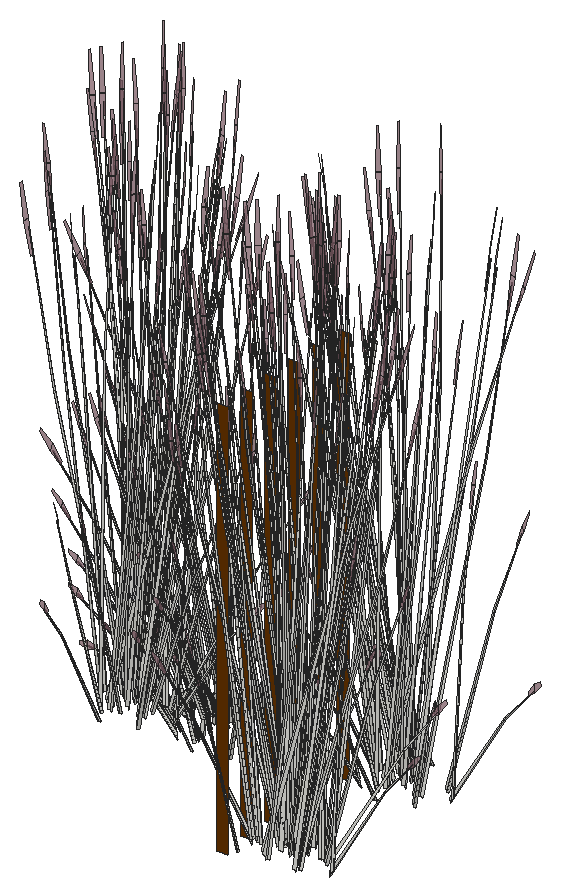
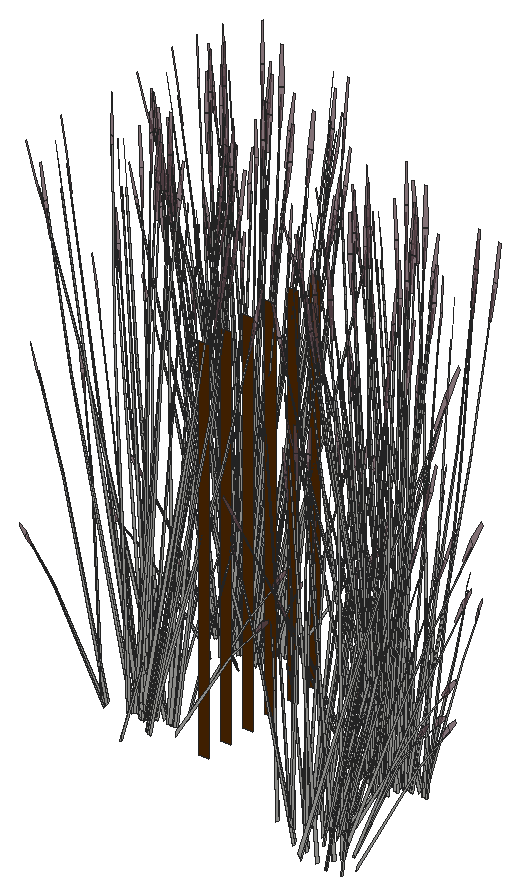
# SketchUp Ruby script. Lengths in inches.
U = 1.inch
M = Sketchup.active_model
def pt(a) = Geom::Point3d.new(a.map { |v| v * U })
def face(e, loops, mat)
  f = e.add_face(loops[0].map { |a| pt(a) })
  loops[1..].each { |l| e.add_face(l.map { |a| pt(a) }).erase! }
  f.material = f.back_material = mat if mat
  f
end
# faces: each face lists its corners as indices into pts; further lists are holes
def faces(e, pts, list, mat = nil) = list.each { |f| face(e, (f[0].is_a?(Array) ? f : [f]).map { |l| l.map { |i| pts[i] } }, mat) }
# xy, xz, yz: faces in a plane at the given z, y or x. An outline is a flat list of corners, or four numbers for a rectangle; further outlines are holes
def ring(l) = l.size == 4 ? [[l[0], l[1]], [l[2], l[1]], [l[2], l[3]], [l[0], l[3]]] : l.each_slice(2).to_a
def flat(e, list, mat, &to3) = list.each { |f| face(e, (f[0].is_a?(Array) ? f : [f]).map { |l| ring(l).map { |u, v| to3.(u, v) } }, mat) }
def xy(e, z, list, mat = nil) = flat(e, list, mat) { |x, y| [x, y, z] }
def xz(e, y, list, mat = nil) = flat(e, list, mat) { |x, z| [x, y, z] }
def yz(e, x, list, mat = nil) = flat(e, list, mat) { |y, z| [x, y, z] }
def lines(e, pts, list) = list.each { |a, b| e.add_line(pt(pts[a]), pt(pts[b])) }
# prism: a flat outline (further loops are holes) pulled along v
def prism(e, loops, v, mat = nil)
  f = face(e, loops, mat); d = Geom::Vector3d.new(v.map { |x| x * U })
  f.pushpull(f.normal.samedirection?(d) ? d.length : -d.length)
end
def box(e, o, s, mat = nil) = prism(e, [[o, [o[0] + s[0], o[1], o[2]], [o[0] + s[0], o[1] + s[1], o[2]], [o[0], o[1] + s[1], o[2]]]], [0, 0, s[2]], mat)
def at(x, y, z, deg = 0) = Geom::Transformation.translation(pt([x, y, z])) * Geom::Transformation.rotation(ORIGIN, Z_AXIS, deg.degrees)
def axes(o, x, y, z) = Geom::Transformation.new([*x, 0, *y, 0, *z, 0, *pt(o).to_a, 1])
def part(name) = M.definitions.add(name)
# library, detail: a bought-in or finely detailed component or shape, given as its bounding box
def library(name, o, s) = part(name).tap { |d| box(d.entities, o, s) }
def detail(e, o, s) = box(e.add_group.entities, o, s)
def put(e, d, t, mat = nil) = e.add_instance(d, t).tap { |i| i.material = mat if mat }
def group(e, t, mat = nil) = e.add_group.tap { |g| g.transformation = t; g.material = mat if mat }.entities
root = M.entities
M.materials.add("C08_Toffee_Ember").color = [102, 51, 0]
M.materials.add("LightPink_Translucent").color = [144, 107, 117]
M.materials["LightPink_Translucent"].alpha = 0.75
c1 = part("blade")
p = [[2.15,0.21,22],[0,0.17,0],[0.09,0.45,0],[2.18,0.31,22],[2.29,0.31,22],[0.38,0.45,0],
  [2.48,0.24,33],[2.49,0.24,33],[2.48,0.22,33]]
faces(c1.entities,p,[[0,1,2,3],[4,5,2,3],[6,3,4,7],[8,0,3,6]])
c2 = part("seeds")
p = [[0.3,-0.1,1.38],[-0.01,-0.03,1.59],[-0.01,-0.03,0.03],[0.14,-0.07,-0.07],[0.29,-0.03,3],[0.15,0.01,3.11]]
faces(c2.entities,p,[[0,1,2,3],[1,0,4,5]],"LightPink_Translucent")
c3 = part("blade with seeds")
put(c3.entities,c1,at(0,0,0))
put(c3.entities,c2,axes([2.4,0.25,30.99],[1.5799,-0.05474,1.17369],[-0.12525,1.92788,0.29478],[-0.07173,-0.02425,1.56792]))
xz(root,322.2,[[693.41,510,694.41,546]],"C08_Toffee_Ember")
xz(root,324.9,[[693.41,510,694.41,546]],"C08_Toffee_Ember")
xz(root,327.6,[[693.41,510,694.41,546]],"C08_Toffee_Ember")
xz(root,330.3,[[693.41,510,694.41,546]],"C08_Toffee_Ember")
xz(root,333,[[693.41,510,694.41,546]],"C08_Toffee_Ember")
xz(root,335.7,[[693.41,510,694.41,546]],"C08_Toffee_Ember")
put(root,c3,axes([697.01,322.31,511.68],[0.45414,-0.35624,-0.25712],[0.45414,0.35624,0.25712],[0,-0.11474,1.15348]))
put(root,c3,axes([696.82,320.6,511.77],[-0.18768,0.46622,-0.03231],[-0.57763,-0.14342,-0.14649],[-0.0877,-0.07626,0.48318]))
put(root,c3,axes([698.6,322.96,512.21],[-0.73268,-0.27244,-0.24149],[0.35279,-0.57501,-0.41502],[-0.02303,-0.14118,1.32557]))
put(root,c3,axes([696.51,322.73,511.97],[-0.81352,0,0],[0,-0.63814,-0.42834],[0,-0.14534,1.3588]))
put(root,c3,axes([698.86,320.83,511.68],[0.60696,0.14127,-0.25712],[-0.15283,0.49751,0.25712],[0.12236,-0.05737,1.15348]))
put(root,c3,axes([697.14,322.56,511.93],[-0.60515,0.48003,0.25528],[-0.60552,-0.47498,-0.30288],[-0.02113,-0.13632,1.36855]))
put(root,c3,axes([699.07,322.78,512.02],[0.73304,0.27674,0.19974],[-0.35279,0.57501,0.41502],[0,-0.13255,1.3325]))
put(root,c3,axes([698.78,323.56,512.02],[0.17244,-0.67657,-0.19446],[0.81759,0.11793,0.42555],[-0.14286,-0.09343,1.29846]))
put(root,c3,axes([701.16,320.84,511.97],[0.40676,-0.57214,0],[0.68052,0.31907,-0.42834],[0.15499,0.07267,1.3588]))
put(root,c3,axes([698.72,323.29,511.83],[-0.39083,-0.47924,-0.37133],[0.59199,-0.33747,0.17871],[-0.12647,-0.0593,1.19224]))
put(root,c3,axes([698.8,322.61,511.96],[0.28286,0.63846,0.37976],[-0.80821,0.22202,0.14902],[0.00988,-0.11732,1.31851]))
put(root,c3,axes([702.76,323.1,511.65],[-0.41902,0.06852,1.17514],[-0.0667,-0.54541,0.06726],[0.29348,-0.08255,0.6687]))
put(root,c3,axes([703.52,322.62,511.875],[-0.40335,-0.3651,-0.05385],[0.44175,-0.33453,-0.24415],[0.12517,-0.02355,0.8053]))
put(root,c3,axes([699.82,322.66,511.83],[0,-0.66065,0],[0.81352,0,0],[0,0,1.48949]))
put(root,c3,axes([698.37,323.47,511.71],[-0.67676,-0.09361,-0.51753],[0.14281,-0.57742,-0.13583],[-0.20196,-0.06997,1.14236]))
put(root,c3,axes([699.4375,322.25,511.96],[-0.53943,0.51816,0.37976],[-0.64086,-0.4574,0.14902],[0.13005,-0.05171,1.31851]))
put(root,c3,axes([700.03,323.17,511.91],[-0.60515,-0.49144,-0.05089],[0.60552,-0.49174,0],[-0.02113,-0.01716,1.45724]))
put(root,c3,axes([698.22,321.85,511.32],[-0.64037,0.22859,1.07011],[-0.20382,-0.65589,0.4158],[0.39323,0.01091,1.21713]))
put(root,c3,axes([699.9375,322.02,512.17],[0.12551,-0.50956,0.12018],[0.6132,0.08845,-0.34318],[0.1116,0.05232,1.05198]))
put(root,c3,axes([698.875,323.23,511.96],[0.82229,0.1203,0.37976],[-0.16734,0.67942,0.14902],[-0.12017,-0.06561,1.31851]))
put(root,c3,axes([703.22,322.74,511.24],[-0.034,-0.08668,1.46364],[0.23582,-0.50706,-0.2236],[0.23788,-0.00729,0.24931]))
put(root,c3,axes([696.2,322.65,511.24],[0.0165,0.08998,1.46364],[-0.33262,0.46992,-0.2236],[-0.23626,-0.02369,0.24931]))
put(root,c3,axes([697.65,324.35,511.68],[-0.15283,-0.49751,-0.25712],[0.60696,-0.14127,0.25712],[-0.12236,-0.05737,1.15348]))
put(root,c3,axes([699.875,322.1875,512.21],[0.65687,-0.37907,-0.24149],[0.43681,0.53562,-0.41502],[0.16207,0.0544,1.32557]))
put(root,c3,axes([697.48,324.5625,511.67],[-0.60889,-0.28548,-0.4121],[0.36394,-0.51192,0],[-0.13868,-0.06502,1.30728]))
put(root,c3,axes([701.53,321.18,511.67],[0.60889,0.28548,-0.4121],[-0.36394,0.51192,0],[0.13868,0.06502,1.30728]))
put(root,c3,axes([700.375,322.81,511.83],[0.72788,0,0],[0,0.59111,0],[0,0,1.48078]))
put(root,c3,axes([699.14,323.55,512.21],[-0.65687,0.37907,-0.24149],[-0.43681,-0.53562,-0.41502],[-0.16207,-0.0544,1.32557]))
put(root,c3,axes([701.36,321.39,511.68],[0.15283,0.49751,-0.25712],[-0.60696,0.14127,0.25712],[0.12236,0.05737,1.15348]))
put(root,c3,axes([700.14,322.51,511.98],[-0.82229,-0.1203,0.40835],[0.16734,-0.67942,0.16024],[0.12017,0.06561,1.41775]))
put(root,c3,axes([699.48,324.1875,511.83],[-0.21227,-0.49226,0],[0.60616,-0.17239,0],[0,0,1.28128]))
put(root,c3,axes([699.08,323.72,512.17],[-0.12551,0.50956,0.12018],[-0.6132,-0.08845,-0.34318],[-0.1116,-0.05232,1.05198]))
put(root,c3,axes([700.28,324.12,511.8125],[0.68303,-0.19373,-0.15934],[0.24001,0.55805,0.00007],[0.07539,-0.02141,1.44335]))
put(root,c3,axes([700.36,323.0625,511.84],[0.45414,0.3688,0],[-0.45414,0.3688,0],[0,0,1.40491]))
put(root,c3,axes([700.64,322.27,511.71],[0.67676,0.09361,-0.51753],[-0.14281,0.57742,-0.13583],[0.20196,0.06997,1.14236]))
put(root,c3,axes([699.33,324.41,511.82],[-0.65588,-0.25634,0],[0.31565,-0.53263,0],[0,0,1.35047]))
put(root,c3,axes([699.88,323.73,512.05],[-0.63528,-0.45956,-0.20909],[0.53456,-0.51604,0.45758],[-0.17107,0.05376,1.39619]))
put(root,c3,axes([700.23,322.93,511.9],[0,0.66033,-0.04679],[-0.81352,0,0],[0,0.02075,1.48875]))
put(root,c3,axes([700.29,322.46,511.83],[0.39083,0.47924,-0.37133],[-0.59199,0.33747,0.17871],[0.12647,0.0593,1.19224]))
put(root,c3,axes([697.86,324.91,511.97],[-0.40676,0.57214,0],[-0.68052,-0.31907,-0.42834],[-0.15499,-0.07267,1.3588]))
put(root,c3,axes([700.625,322.75,512.17],[0.60616,-0.16651,0.12018],[0.21227,0.47548,-0.34318],[0,0.10465,1.05198]))
put(root,c3,axes([699.56,323.63,511.83],[-0.70648,0.03525,-0.37133],[-0.06389,-0.58508,0.17871],[-0.12647,0.0593,1.19224]))
put(root,c3,axes([700.08,324.42,511.83],[0.65588,0.25634,0],[-0.31565,0.53263,0],[0,0,1.45212]))
put(root,c3,axes([700.34,324.99,511.82],[-0.40169,-0.57414,-0.04268],[0.68052,-0.31907,0.42834],[-0.16769,0.05466,1.35813]))
put(root,c3,axes([700.2,323.6,512.17],[0.48065,0.34305,0.12018],[-0.40092,0.38703,-0.34318],[-0.1116,0.05232,1.05198]))
put(root,c3,axes([699.84,324.2,511.9],[0.28286,0.65594,-0.0499],[-0.80821,0.22985,0],[0.00988,0.02291,1.42904]))
put(root,c3,axes([700.16,324.91,511.68],[-0.60696,-0.14127,-0.25712],[0.15283,-0.49751,0.25712],[-0.12236,0.05737,1.15348]))
put(root,c3,axes([702.5,323.02,511.97],[0.81352,0,0],[0,0.63814,-0.42834],[0,0.14534,1.3588]))
put(root,c3,axes([702.18,323.34,511.83],[-0.81312,-0.00457,-0.0413],[0,-0.63814,0.41452],[-0.02555,0.14527,1.31432]))
put(root,c3,axes([700.42,322.79,512.21],[0.73268,0.27244,-0.24149],[-0.35279,0.57501,-0.41502],[0.02303,0.14118,1.32557]))
put(root,c3,axes([702.01,323.4375,511.68],[-0.45414,0.35624,-0.25712],[-0.45414,-0.35624,0.25712],[0,0.11474,1.15348]))
put(root,c3,axes([700.05,323.47,512.21],[0.07581,0.65151,-0.24149],[-0.7896,0.03939,-0.41502],[-0.13904,0.08678,1.32557]))
put(root,c3,axes([678.39,330.45,512.15],[-0.18493,0.11557,1.18691],[-0.55384,-0.20228,-0.25526],[0.10266,-0.25157,0.50747]))
put(root,c3,axes([700.34,323.22,511.83],[-0.31565,0.51449,-0.37133],[-0.65588,-0.24761,0.17871],[0,0.1186,1.19224]))
put(root,c3,axes([677.01,329.83,511.24],[-0.10912,0.02057,1.46364],[-0.60346,-0.23156,-0.2236],[0.01013,-0.19315,0.24931]))
put(root,c3,axes([699.58,323.97,511.71],[-0.43821,0.42916,-0.51753],[-0.54436,-0.38915,-0.13583],[-0.1756,0.10706,1.14236]))
put(root,c3,axes([700.36,324.69,511.93],[0.81449,0.18558,0.25528],[-0.20377,0.66335,-0.30288],[-0.13481,0.08302,1.36855]))
put(root,c3,axes([700.3,325.14,511.67],[-0.60889,0.28548,-0.4121],[-0.36394,-0.51192,0],[-0.13868,0.06502,1.30728]))
put(root,c3,axes([702.32,323.45,511.67],[0,0.57097,-0.4121],[-0.72788,0,0],[0,0.13004,1.30728]))
put(root,c3,axes([700.85,325.05,511.97],[0.40676,0.57214,0],[-0.68052,0.31907,-0.42834],[-0.15499,0.07267,1.3588]))
put(root,c3,axes([701.5,325.24,511.24],[0.0474,-0.08243,1.46364],[0.59674,-0.24277,-0.2236],[0.18092,0.12565,0.24931]))
put(root,c3,axes([700.71,323.37,511.74],[0.23855,0.52277,-0.57446],[-0.68718,0.18827,-0.15077],[0.02637,0.17702,1.26801]))
put(root,c3,axes([696.02,325.17,511.24],[0.08727,0.05704,1.46364],[0.14797,0.52853,-0.2236],[-0.19341,0.11271,0.24931]))
put(root,c3,axes([676.11,332.6,511.74],[-0.26718,-0.5855,-0.57963],[0.76964,-0.21087,-0.15213],[-0.02953,-0.19827,1.27944]))
put(root,c3,axes([679.68,330.8125,511.24],[-0.09738,-0.04498,1.46364],[-0.25012,-0.50252,-0.2236],[0.16873,-0.13637,0.24931]))
put(root,c3,axes([698.71,325.23,511.24],[0.10529,-0.03107,1.46364],[0.63335,0.17101,-0.2236],[0.01852,0.19274,0.24931]))
put(root,c3,axes([676,330.92,511.97],[-0.40676,-0.57214,0],[0.68052,-0.31907,-0.42834],[0.15499,-0.07267,1.3588]))
put(root,c3,axes([676.9,330.23,511.77],[-0.44958,0.32756,-0.03231],[-0.41194,-0.35875,-0.14649],[-0.029,-0.10165,0.48318]))
put(root,c3,axes([697.26,325.3,512.34],[0.59102,-0.10111,0.05401],[0.13587,0.40735,-0.71633],[-0.03747,0.2062,0.64209]))
put(root,c3,axes([674.53,332.52,511.67],[0,-0.57097,-0.4121],[0.72788,0,0],[0,-0.13004,1.30728]))
put(root,c3,axes([676.55,330.83,511.67],[0.60889,-0.28548,-0.4121],[0.36394,0.51192,0],[0.13868,-0.06502,1.30728]))
put(root,c3,axes([680.17,331.8125,512.15],[-0.23242,-0.01691,1.18691],[-0.23811,-0.45367,-0.25526],[0.28553,-0.12834,0.50747]))
put(root,c3,axes([677.28,332,511.71],[0.43821,-0.42916,-0.51753],[0.54436,0.38915,-0.13583],[0.1756,-0.10706,1.14236]))
put(root,c3,axes([699.17,333.1,511.24],[-0.10912,0.02057,1.46364],[-0.60346,-0.23156,-0.2236],[0.01013,-0.19315,0.24931]))
put(root,c3,axes([676.51,332.75,511.83],[0.31565,-0.51449,-0.37133],[0.65588,0.24761,0.17871],[0,-0.1186,1.19224]))
put(root,c3,axes([676.8,332.5,512.21],[-0.07581,-0.65151,-0.24149],[0.7896,-0.03939,-0.41502],[0.13904,-0.08678,1.32557]))
put(root,c3,axes([674.84,332.53,511.68],[0.45414,-0.35624,-0.25712],[0.45414,0.35624,0.25712],[0,-0.11474,1.15348]))
put(root,c3,axes([676.43,333.18,512.21],[-0.73268,-0.27244,-0.24149],[0.35279,-0.57501,-0.41502],[-0.02303,-0.14118,1.32557]))
put(root,c3,axes([676.7,331.05,511.68],[0.60696,0.14127,-0.25712],[-0.15283,0.49751,0.25712],[0.12236,-0.05737,1.15348]))
put(root,c3,axes([676.9,333.01,512.02],[0.73304,0.27674,0.19974],[-0.35279,0.57501,0.41502],[0,-0.13255,1.3325]))
put(root,c3,axes([697.22,333.81,511.24],[-0.06302,0.07522,1.46364],[-0.63686,0.16217,-0.2236],[-0.15385,-0.14752,0.24931]))
put(root,c3,axes([698.27,335.875,511.74],[-0.26718,-0.5855,-0.57963],[0.76964,-0.21087,-0.15213],[-0.02953,-0.19827,1.27944]))
put(root,c3,axes([701.84,334.09,511.24],[-0.09738,-0.04498,1.46364],[-0.25012,-0.50252,-0.2236],[0.16873,-0.13637,0.24931]))
put(root,c3,axes([679,331.0625,511.97],[0.40676,-0.57214,0],[0.68052,0.31907,-0.42834],[0.15499,0.07267,1.3588]))
put(root,c3,axes([676.64,332.83,511.96],[0.28286,0.63846,0.37976],[-0.80821,0.22202,0.14902],[0.00988,-0.11732,1.31851]))
put(root,c3,axes([680.6,333.32,511.65],[-0.41902,0.06852,1.17514],[-0.0667,-0.54541,0.06726],[0.29348,-0.08255,0.6687]))
put(root,c3,axes([681.36,332.84,511.875],[-0.40335,-0.3651,-0.05385],[0.44175,-0.33453,-0.24415],[0.12517,-0.02355,0.8053]))
put(root,c3,axes([677.66,332.89,511.83],[0,-0.66065,0],[0.81352,0,0],[0,0,1.48949]))
put(root,c3,axes([698.16,334.19,511.97],[-0.40676,-0.57214,0],[0.68052,-0.31907,-0.42834],[0.15499,-0.07267,1.3588]))
put(root,c3,axes([699.06,333.5,511.77],[-0.44958,0.32756,-0.03231],[-0.41194,-0.35875,-0.14649],[-0.029,-0.10165,0.48318]))
put(root,c3,axes([677.28,332.47,511.96],[-0.53943,0.51816,0.37976],[-0.64086,-0.4574,0.14902],[0.13005,-0.05171,1.31851]))
put(root,c3,axes([677.86,333.4,511.91],[-0.60515,-0.49144,-0.05089],[0.60552,-0.49174,0],[-0.02113,-0.01716,1.45724]))
put(root,c3,axes([676.05,332.07,511.32],[-0.64037,0.22859,1.07011],[-0.20382,-0.65589,0.4158],[0.39323,0.01091,1.21713]))
put(root,c3,axes([677.78,332.25,512.17],[0.12551,-0.50956,0.12018],[0.6132,0.08845,-0.34318],[0.1116,0.05232,1.05198]))
put(root,c3,axes([676.71,333.46,511.96],[0.82229,0.1203,0.37976],[-0.16734,0.67942,0.14902],[-0.12017,-0.06561,1.31851]))
put(root,c3,axes([681.06,332.97,511.24],[-0.034,-0.08668,1.46364],[0.23582,-0.50706,-0.2236],[0.23788,-0.00729,0.24931]))
put(root,c3,axes([696.69,335.79,511.67],[0,-0.57097,-0.4121],[0.72788,0,0],[0,-0.13004,1.30728]))
put(root,c3,axes([698.72,334.1,511.67],[0.60889,-0.28548,-0.4121],[0.36394,0.51192,0],[0.13868,-0.06502,1.30728]))
put(root,c3,axes([699.4375,335.28,511.71],[0.43821,-0.42916,-0.51753],[0.54436,0.38915,-0.13583],[0.1756,-0.10706,1.14236]))
put(root,c3,axes([678.375,337.75,508.64],[0.14872,0.18332,1.42242],[-0.6872,0.15433,0.11501],[-0.15531,-0.28779,0.60807]))
put(root,c3,axes([677.71,332.41,512.21],[0.65687,-0.37907,-0.24149],[0.43681,0.53562,-0.41502],[0.16207,0.0544,1.32557]))
put(root,c3,axes([679.51,336.54,509.34],[-0.09951,-0.08005,1.45204],[-0.66407,0.05075,-0.22964],[-0.10598,-0.19148,0.11645]))
put(root,c3,axes([681.05,337.49,507.57],[-0.18493,0.11557,1.18691],[-0.55384,-0.20228,-0.25526],[0.10266,-0.25157,0.50747]))
put(root,c3,axes([679.37,331.41,511.67],[0.60889,0.28548,-0.4121],[-0.36394,0.51192,0],[0.13868,0.06502,1.30728]))
put(root,c3,axes([680.21,337.89,509.56],[-0.31051,-0.46426,-0.58968],[0.63919,-0.25873,0.07116],[-0.07261,-0.22432,0.83415]))
put(root,c3,axes([678.21,333.03,511.83],[0.72788,0,0],[0,0.59111,0],[0,0,1.48078]))
put(root,c3,axes([698.67,336.03,511.83],[0.31565,-0.51449,-0.37133],[0.65588,0.24761,0.17871],[0,-0.1186,1.19224]))
put(root,c3,axes([678.1875,337.27,507.57],[-0.0394,0.18678,1.18691],[-0.57594,0.15636,-0.25526],[-0.13463,-0.24142,0.50747]))
put(root,c3,axes([698.96,335.77,512.21],[-0.07581,-0.65151,-0.24149],[0.7896,-0.03939,-0.41502],[0.13904,-0.08678,1.32557]))
put(root,c3,axes([697.01,335.81,511.68],[0.45414,-0.35624,-0.25712],[0.45414,0.35624,0.25712],[0,-0.11474,1.15348]))
put(root,c3,axes([679.67,336.86,506.66],[-0.10912,0.02057,1.46364],[-0.60346,-0.23156,-0.2236],[0.01013,-0.19315,0.24931]))
put(root,c3,axes([696.82,334.1,511.77],[-0.18768,0.46622,-0.03231],[-0.57763,-0.14342,-0.14649],[-0.0877,-0.07626,0.48318]))
put(root,c3,axes([698.6,336.46,512.21],[-0.73268,-0.27244,-0.24149],[0.35279,-0.57501,-0.41502],[-0.02303,-0.14118,1.32557]))
put(root,c3,axes([679.2,331.62,511.68],[0.15283,0.49751,-0.25712],[-0.60696,0.14127,0.25712],[0.12236,0.05737,1.15348]))
put(root,c3,axes([696.51,336.23,511.97],[-0.81352,0,0],[0,-0.63814,-0.42834],[0,-0.14534,1.3588]))
put(root,c3,axes([681.5,338.35,509.56],[0.01693,-0.52814,-0.58968],[0.71285,0.03547,0.07116],[0.07523,-0.22375,0.83415]))
put(root,c3,axes([698.86,334.33,511.68],[0.60696,0.14127,-0.25712],[-0.15283,0.49751,0.25712],[0.12236,-0.05737,1.15348]))
put(root,c3,axes([677.98,332.73,511.98],[-0.82229,-0.1203,0.40835],[0.16734,-0.67942,0.16024],[0.12017,0.06561,1.41775]))
put(root,c3,axes([677.32,334.41,511.83],[-0.21227,-0.49226,0],[0.60616,-0.17239,0],[0,0,1.28128]))
put(root,c3,axes([682.49,337.52,509.34],[-0.00628,-0.11364,1.45204],[-0.53042,-0.32843,-0.22964],[0.08201,-0.19909,0.11645]))
put(root,c3,axes([680.27,337.5,509.18],[0.19614,-0.43908,-0.29394],[0.57222,0.12807,0.37948],[-0.05247,-0.17678,0.72609]))
put(root,c3,axes([680.7,338.08,508.64],[-0.12114,0.19625,1.42242],[-0.50818,-0.40613,0.11501],[0.22925,-0.25313,0.60807]))
put(root,c3,axes([682.35,337.11,509.33],[-0.06607,0.04361,1.47228],[-0.64734,-0.14714,-0.13912],[-0.02343,-0.19032,0.26054]))
put(root,c3,axes([678.12,334.34,511.8125],[0.68303,-0.19373,-0.15934],[0.24001,0.55805,0.00007],[0.07539,-0.02141,1.44335]))
put(root,c3,axes([678.2,333.29,511.84],[0.45414,0.3688,0],[-0.45414,0.3688,0],[0,0,1.40491]))
put(root,c3,axes([679.97,337.8,509.31],[-0.63954,-0.14313,-0.42412],[0.21921,-0.49074,-0.32852],[-0.05864,-0.19758,0.81151]))
put(root,c3,axes([680.37,336.57,507.72],[0.08346,0.33295,0.95334],[-0.46298,-0.1844,0.70045],[0.04982,-0.17048,0.20998]))
put(root,c3,axes([681.36,338.17,509.31],[-0.46573,-0.38364,-0.42412],[0.49199,-0.33598,-0.32852],[0.07086,-0.19492,0.81151]))
put(root,c3,axes([678.48,332.5,511.71],[0.67676,0.09361,-0.51753],[-0.14281,0.57742,-0.13583],[0.20196,0.06997,1.14236]))
put(root,c3,axes([678.83,336.28,509.33],[-0.01214,0.06844,1.47228],[-0.59861,0.24837,-0.13912],[-0.17615,-0.12696,0.26054]))
put(root,c3,axes([677.17,334.63,511.82],[-0.65588,-0.25634,0],[0.31565,-0.53263,0],[0,0,1.35047]))
put(root,c3,axes([697.14,336.06,511.93],[-0.60515,0.48003,0.25528],[-0.60552,-0.47498,-0.30288],[-0.02113,-0.13632,1.36855]))
put(root,c3,axes([678.7,337.49,509.65],[0.72473,-0.14676,0.44623],[0.12578,0.57568,0.36794],[-0.17045,-0.16967,0.92337]))
put(root,c3,axes([699.07,336.28,512.02],[0.73304,0.27674,0.19974],[-0.35279,0.57501,0.41502],[0,-0.13255,1.3325]))
put(root,c3,axes([698.78,337.06,512.02],[0.17244,-0.67657,-0.19446],[0.81759,0.11793,0.42555],[-0.14286,-0.09343,1.29846]))
put(root,c3,axes([680.34,337.6,509.35],[0.64106,0.14927,0.39842],[-0.21921,0.49074,0.32852],[-0.03852,-0.19299,0.82444]))
put(root,c3,axes([680.52,337.77,509.6],[-0.63664,0.26583,-0.10093],[-0.31286,-0.47181,-0.56021],[-0.084,-0.19882,0.85122]))
put(root,c3,axes([678.07,333.15,511.9],[0,0.66033,-0.04679],[-0.81352,0,0],[0,0.02075,1.48875]))
put(root,c3,axes([681.84,338.37,509.6],[-0.71502,-0.02829,-0.10093],[0.01954,-0.53563,-0.56021],[0.04967,-0.20629,0.85122]))
put(root,c3,axes([681.79,338.03,509.18],[0.4402,-0.30062,-0.29394],[0.41671,0.34326,0.37948],[0.0634,-0.1744,0.72609]))
put(root,c3,axes([677.99,336.97,507.72],[0.33937,0.19872,0.95334],[-0.49424,0.11946,0.70045],[-0.10575,-0.15273,0.20998]))
put(root,c3,axes([678.13,332.68,511.83],[0.39083,0.47924,-0.37133],[-0.59199,0.33747,0.17871],[0.12647,0.0593,1.19224]))
put(root,c3,axes([680.51,337.5625,509.35],[0.47939,-0.19405,0.05337],[0.23464,0.35385,0.42015],[-0.0463,-0.15598,0.64067]))
put(root,c3,axes([678.62,337.66,509.18],[-0.10048,-0.4599,-0.29394],[0.5744,-0.12144,0.37948],[-0.15428,-0.13179,0.72609]))
put(root,c3,axes([678.46,332.97,512.17],[0.60616,-0.16651,0.12018],[0.21227,0.47548,-0.34318],[0,0.10465,1.05198]))
put(root,c3,axes([701.16,334.34,511.97],[0.40676,-0.57214,0],[0.68052,0.31907,-0.42834],[0.15499,0.07267,1.3588]))
put(root,c3,axes([698.72,336.79,511.83],[-0.39083,-0.47924,-0.37133],[0.59199,-0.33747,0.17871],[-0.12647,-0.0593,1.19224]))
put(root,c3,axes([698.8,336.11,511.96],[0.28286,0.63846,0.37976],[-0.80821,0.22202,0.14902],[0.00988,-0.11732,1.31851]))
put(root,c3,axes([680.72,334.13,512.15],[-0.15668,-0.14043,1.18691],[0.20386,-0.46454,-0.25526],[0.31701,0.06293,0.50747]))
put(root,c3,axes([678.87,337.62,509.35],[0.29569,-0.36271,0.05337],[0.42107,0.21117,0.42015],[-0.13613,-0.11629,0.64067]))
put(root,c3,axes([677.72,337.57,506.66],[-0.06302,0.07522,1.46364],[-0.63686,0.16217,-0.2236],[-0.15385,-0.14752,0.24931]))
put(root,c3,axes([702.76,336.6,511.65],[-0.41902,0.06852,1.17514],[-0.0667,-0.54541,0.06726],[0.29348,-0.08255,0.6687]))
put(root,c3,axes([703.52,336.12,511.875],[-0.40335,-0.3651,-0.05385],[0.44175,-0.33453,-0.24415],[0.12517,-0.02355,0.8053]))
put(root,c3,axes([677.92,334.64,511.83],[0.65588,0.25634,0],[-0.31565,0.53263,0],[0,0,1.45212]))
put(root,c3,axes([678.77,339.64,507.17],[-0.26718,-0.5855,-0.57963],[0.76964,-0.21087,-0.15213],[-0.02953,-0.19827,1.27944]))
put(root,c3,axes([682.34,337.85,506.66],[-0.09738,-0.04498,1.46364],[-0.25012,-0.50252,-0.2236],[0.16873,-0.13637,0.24931]))
put(root,c3,axes([699.82,336.16,511.83],[0,-0.66065,0],[0.81352,0,0],[0,0,1.48949]))
put(root,c3,axes([678.18,335.21,511.82],[-0.40169,-0.57414,-0.04268],[0.68052,-0.31907,0.42834],[-0.16769,0.05466,1.35813]))
put(root,c3,axes([678.04,333.82,512.17],[0.48065,0.34305,0.12018],[-0.40092,0.38703,-0.34318],[-0.1116,0.05232,1.05198]))
put(root,c3,axes([680.33,337.96,509.62],[-0.19614,0.43908,0.29394],[-0.57222,-0.12807,-0.37948],[-0.05247,-0.17678,0.72609]))
put(root,c3,axes([698.37,336.97,511.71],[-0.67676,-0.09361,-0.51753],[0.14281,-0.57742,-0.13583],[-0.20196,-0.06997,1.14236]))
put(root,c3,axes([699.4375,335.75,511.96],[-0.53943,0.51816,0.37976],[-0.64086,-0.4574,0.14902],[0.13005,-0.05171,1.31851]))
put(root,c3,axes([681.79,338.14,509.35],[0.46327,0.38957,0.39842],[-0.49199,0.33598,0.32852],[0.08546,-0.18277,0.82444]))
put(root,c3,axes([681.96,338.18,509.35],[0.53464,0.0266,0.05337],[-0.01466,0.40172,0.42015],[0.05594,-0.15388,0.64067]))
put(root,c3,axes([700.03,336.67,511.91],[-0.60515,-0.49144,-0.05089],[0.60552,-0.49174,0],[-0.02113,-0.01716,1.45724]))
put(root,c3,axes([681.5625,338.45,509.62],[-0.4402,0.30062,0.29394],[-0.41671,-0.34326,-0.37948],[0.0634,-0.1744,0.72609]))
put(root,c3,axes([679.375,340.13,512.15],[-0.18493,0.11557,1.18691],[-0.55384,-0.20228,-0.25526],[0.10266,-0.25157,0.50747]))
put(root,c3,axes([682.34,339.26,509.56],[0.33983,-0.45051,-0.58968],[0.59551,0.32017,0.07116],[0.20291,-0.16322,0.83415]))
put(root,c3,axes([698.22,335.35,511.32],[-0.64037,0.22859,1.07011],[-0.20382,-0.65589,0.4158],[0.39323,0.01091,1.21713]))
put(root,c3,axes([678.67,337.95,507.39],[-0.40676,-0.57214,0],[0.68052,-0.31907,-0.42834],[0.15499,-0.07267,1.3588]))
put(root,c3,axes([682.32,339.05,509.31],[-0.16713,-0.52135,-0.42412],[0.63294,-0.0912,-0.32852],[0.18138,-0.14003,0.81151]))
put(root,c3,axes([699.9375,335.52,512.17],[0.12551,-0.50956,0.12018],[0.6132,0.08845,-0.34318],[0.1116,0.05232,1.05198]))
put(root,c3,axes([679.56,337.26,507.19],[-0.44958,0.32756,-0.03231],[-0.41194,-0.35875,-0.14649],[-0.029,-0.10165,0.48318]))
put(root,c3,axes([677.68,334.43,511.9],[0.28286,0.65594,-0.0499],[-0.80821,0.22985,0],[0.00988,0.02291,1.42904]))
put(root,c3,axes([698.875,336.73,511.96],[0.82229,0.1203,0.37976],[-0.16734,0.67942,0.14902],[-0.12017,-0.06561,1.31851]))
put(root,c3,axes([677.99,335.14,511.68],[-0.60696,-0.14127,-0.25712],[0.15283,-0.49751,0.25712],[-0.12236,0.05737,1.15348]))
put(root,c3,axes([703.22,336.24,511.24],[-0.034,-0.08668,1.46364],[0.23582,-0.50706,-0.2236],[0.23788,-0.00729,0.24931]))
put(root,c3,axes([696.2,336.15,511.24],[0.0165,0.08998,1.46364],[-0.33262,0.46992,-0.2236],[-0.23626,-0.02369,0.24931]))
put(root,c3,axes([678,339.5,511.24],[-0.10912,0.02057,1.46364],[-0.60346,-0.23156,-0.2236],[0.01013,-0.19315,0.24931]))
put(root,c3,axes([699.17,339.5,511.24],[-0.10912,0.02057,1.46364],[-0.60346,-0.23156,-0.2236],[0.01013,-0.19315,0.24931]))
put(root,c3,axes([680.34,333.24,511.97],[0.81352,0,0],[0,0.63814,-0.42834],[0,0.14534,1.3588]))
put(root,c3,axes([682.62,339.43,509.6],[-0.60181,-0.31483,-0.10093],[0.34671,-0.45593,-0.56021],[0.17003,-0.15849,0.85122]))
put(root,c3,axes([680.02,333.57,511.83],[-0.81312,-0.00457,-0.0413],[0,-0.63814,0.41452],[-0.02555,0.14527,1.31432]))
put(root,c3,axes([697.65,337.85,511.68],[-0.15283,-0.49751,-0.25712],[0.60696,-0.14127,0.25712],[-0.12236,-0.05737,1.15348]))
put(root,c3,axes([678.26,333.01,512.21],[0.73268,0.27244,-0.24149],[-0.35279,0.57501,-0.41502],[0.02303,0.14118,1.32557]))
put(root,c3,axes([679.85,333.66,511.68],[-0.45414,0.35624,-0.25712],[-0.45414,-0.35624,0.25712],[0,0.11474,1.15348]))
put(root,c3,axes([677.89,333.69,512.21],[0.07581,0.65151,-0.24149],[-0.7896,0.03939,-0.41502],[-0.13904,0.08678,1.32557]))
put(root,c3,axes([699.875,335.6875,512.21],[0.65687,-0.37907,-0.24149],[0.43681,0.53562,-0.41502],[0.16207,0.0544,1.32557]))
put(root,c3,axes([680.14,341.15,508.18],[0.56221,0.23024,1.25546],[-0.55078,0.49601,0.49647],[-0.2467,-0.29398,1.05249]))
put(root,c3,axes([678.18,333.44,511.83],[-0.31565,0.51449,-0.37133],[-0.65588,-0.24761,0.17871],[0,0.1186,1.19224]))
put(root,c3,axes([678.96,338.03,509.62],[0.10048,0.4599,0.29394],[-0.5744,0.12144,-0.37948],[-0.15428,-0.13179,0.72609]))
put(root,c3,axes([697.48,338.0625,511.67],[-0.60889,-0.28548,-0.4121],[0.36394,-0.51192,0],[-0.13868,-0.06502,1.30728]))
put(root,c3,axes([677.2,339.55,507.1],[0,-0.57097,-0.4121],[0.72788,0,0],[0,-0.13004,1.30728]))
put(root,c3,axes([701.53,334.68,511.67],[0.60889,0.28548,-0.4121],[-0.36394,0.51192,0],[0.13868,0.06502,1.30728]))
put(root,c3,axes([679.22,337.86,507.1],[0.60889,-0.28548,-0.4121],[0.36394,0.51192,0],[0.13868,-0.06502,1.30728]))
put(root,c3,axes([682.83,338.85,507.57],[-0.23242,-0.01691,1.18691],[-0.23811,-0.45367,-0.25526],[0.28553,-0.12834,0.50747]))
put(root,c3,axes([684.1,339.29,509.33],[-0.08498,-0.00434,1.47228],[-0.35287,-0.46464,-0.13912],[0.14171,-0.15278,0.26054]))
put(root,c3,axes([700.375,336.31,511.83],[0.72788,0,0],[0,0.59111,0],[0,0,1.48078]))
put(root,c3,axes([699.14,337.05,512.21],[-0.65687,0.37907,-0.24149],[-0.43681,-0.53562,-0.41502],[-0.16207,-0.0544,1.32557]))
put(root,c3,axes([679.94,339.03,507.13],[0.43821,-0.42916,-0.51753],[0.54436,0.38915,-0.13583],[0.1756,-0.10706,1.14236]))
